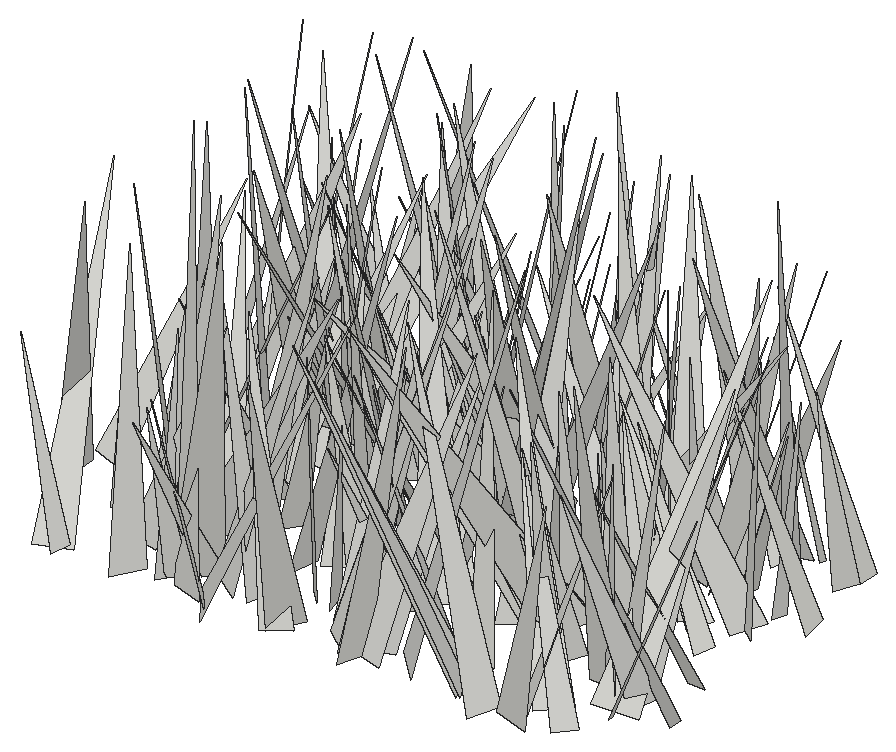
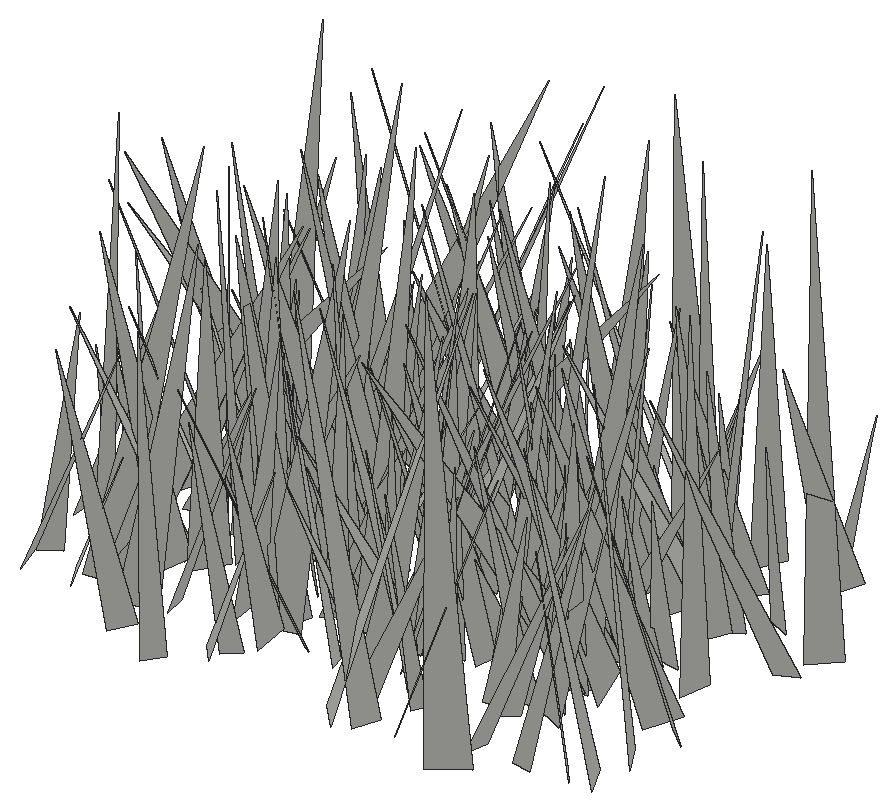
# SketchUp Ruby script. Lengths in inches.
U = 1.inch
M = Sketchup.active_model
def pt(a) = Geom::Point3d.new(a.map { |v| v * U })
def face(e, loops, mat)
  f = e.add_face(loops[0].map { |a| pt(a) })
  loops[1..].each { |l| e.add_face(l.map { |a| pt(a) }).erase! }
  f.material = f.back_material = mat if mat
  f
end
# faces: each face lists its corners as indices into pts; further lists are holes
def faces(e, pts, list, mat = nil) = list.each { |f| face(e, (f[0].is_a?(Array) ? f : [f]).map { |l| l.map { |i| pts[i] } }, mat) }
# xy, xz, yz: faces in a plane at the given z, y or x. An outline is a flat list of corners, or four numbers for a rectangle; further outlines are holes
def ring(l) = l.size == 4 ? [[l[0], l[1]], [l[2], l[1]], [l[2], l[3]], [l[0], l[3]]] : l.each_slice(2).to_a
def flat(e, list, mat, &to3) = list.each { |f| face(e, (f[0].is_a?(Array) ? f : [f]).map { |l| ring(l).map { |u, v| to3.(u, v) } }, mat) }
def xy(e, z, list, mat = nil) = flat(e, list, mat) { |x, y| [x, y, z] }
def xz(e, y, list, mat = nil) = flat(e, list, mat) { |x, z| [x, y, z] }
def yz(e, x, list, mat = nil) = flat(e, list, mat) { |y, z| [x, y, z] }
def lines(e, pts, list) = list.each { |a, b| e.add_line(pt(pts[a]), pt(pts[b])) }
# prism: a flat outline (further loops are holes) pulled along v
def prism(e, loops, v, mat = nil)
  f = face(e, loops, mat); d = Geom::Vector3d.new(v.map { |x| x * U })
  f.pushpull(f.normal.samedirection?(d) ? d.length : -d.length)
end
def box(e, o, s, mat = nil) = prism(e, [[o, [o[0] + s[0], o[1], o[2]], [o[0] + s[0], o[1] + s[1], o[2]], [o[0], o[1] + s[1], o[2]]]], [0, 0, s[2]], mat)
def at(x, y, z, deg = 0) = Geom::Transformation.translation(pt([x, y, z])) * Geom::Transformation.rotation(ORIGIN, Z_AXIS, deg.degrees)
def axes(o, x, y, z) = Geom::Transformation.new([*x, 0, *y, 0, *z, 0, *pt(o).to_a, 1])
def part(name) = M.definitions.add(name)
# library, detail: a bought-in or finely detailed component or shape, given as its bounding box
def library(name, o, s) = part(name).tap { |d| box(d.entities, o, s) }
def detail(e, o, s) = box(e.add_group.entities, o, s)
def put(e, d, t, mat = nil) = e.add_instance(d, t).tap { |i| i.material = mat if mat }
def group(e, t, mat = nil) = e.add_group.tap { |g| g.transformation = t; g.material = mat if mat }.entities
root = M.entities
c1 = part("fur_instance\#9")
p = [[0.8125,0,1.79],[0.67,-0.02,1.48],[0,-0.11,0],[0,0.11,0]]
faces(c1.entities,p,[[0,1,2,3]])
put(root,c1,axes([122.97,12.12,-27.1],[4.57924,-4.33247,0.58798],[-4.22206,-4.60304,-1.03525],[-1.13589,-0.35667,6.21836]))
put(root,c1,axes([129.89,12.79,-27.1],[-6.83596,-2.73328,0.53057],[-2.58478,6.75268,1.48423],[1.035,-1.18879,7.21098]))
put(root,c1,axes([132.79,11.72,-27.1],[0.54307,-5.39112,1.14857],[-5.29865,-0.1925,1.60174],[1.51911,1.25582,5.17624]))
put(root,c1,axes([129.98,12.7,-27.1],[-5.72076,-3.26575,0.35826],[-3.1922,5.6955,0.94426],[0.77675,-0.64548,6.51924]))
put(root,c1,axes([118.09,12.47,-27.1],[2.18541,-3.04998,0.78828],[-3.02604,-2.29919,-0.50659],[-0.87571,0.3334,3.71777]))
put(root,c1,axes([118.98,13.31,-27.1],[1.51991,-3.61395,0.26794],[-3.4425,-1.53065,-1.11749],[-1.13207,-0.1975,3.75792]))
put(root,c1,axes([113.92,11.49,-27.1],[-3.79892,0.58903,0.61511],[0.5899,3.84804,-0.04166],[0.61427,-0.05255,3.84409]))
put(root,c1,axes([126.1,11.77,-27.1],[6.14943,-1.42717,1.61929],[-1.52874,-6.3314,0.22535],[-1.52376,0.59247,6.30885]))
put(root,c1,axes([118.09,13.56,-27.1],[6.18232,-5.30847,0.7026],[-5.32058,-6.21081,-0.10875],[-0.60412,0.37485,8.14795]))
put(root,c1,axes([119.89,11.47,-27.1],[5.9079,4.20697,0.32991],[4.15488,-5.69984,-1.72033],[0.73785,-1.5887,7.04573]))
put(root,c1,axes([120.04,11.49,-27.1],[-3.12705,-1.8127,0.50032],[-1.87769,2.95706,-1.02213],[-0.10232,1.13341,3.46693]))
put(root,c1,axes([116.66,11.66,-27.1],[-5.0872,2.66073,2.45988],[2.85923,5.55214,-0.09239],[2.22604,-1.05084,5.74025]))
put(root,c1,axes([122.9,11.67,-27.1],[-2.01026,5.06538,1.49078],[5.275,1.85579,0.80751],[-0.23431,-1.67916,5.38954]))
put(root,c1,axes([131.7,11.64,-27.1],[-6.69944,1.03913,0.45559],[1.00559,6.70154,-0.49804],[0.5255,0.42362,6.76123]))
put(root,c1,axes([125.62,12.28,-27.1],[5.24089,-0.83273,1.62957],[-1.05437,-5.41429,0.62423],[-1.49573,0.89885,5.2698]))
put(root,c1,axes([126.2,12.0625,-27.1],[0.11042,6.13884,2.00494],[6.14565,0.51615,-1.91884],[1.98398,-1.94051,5.83229]))
put(root,c1,axes([111.09,15.68,-27.1],[8.00988,-2.00577,0.3429],[-1.833,-7.71682,-2.32157],[-0.88363,-2.17404,7.92412]))
put(root,c1,axes([119.03,11.81,-27.1],[2.99088,7.34321,2.70362],[7.47912,-3.53374,1.32409],[-2.30112,-1.94104,7.81761]))
put(root,c1,axes([134.58,12.33,-27.1],[-1.36293,4.52681,0.55653],[4.38086,1.13777,1.47406],[-1.26877,-0.93423,4.49185]))
put(root,c1,axes([117.8,12.125,-27.1],[-4.10668,0.43412,1.0008],[0.12519,4.05996,-1.24738],[1.0837,1.17608,3.93666]))
put(root,c1,axes([132.625,14.21,-27.1],[1.7038,-4.78318,1.39426],[-4.94528,-1.80274,-0.14134],[-0.60574,1.26373,5.0756]))
put(root,c1,axes([119.65,13,-27.1],[3.29943,5.39851,1.49465],[5.593,-3.07886,-1.22601],[0.31023,-1.9081,6.20701]))
put(root,c1,axes([133.89,15.56,-27.1],[0.64901,-7.30772,0.94418],[-7.33385,-0.54888,0.79295],[0.71332,1.00569,7.2935]))
put(root,c1,axes([132.78,12.3125,-27.1],[3.07177,3.42083,0.35758],[3.42072,-3.08846,0.16062],[-0.35863,-0.15826,4.59478]))
put(root,c1,axes([135.51,15.33,-27.1],[3.42862,-3.42654,1.21049],[-3.04602,-3.61734,-1.61199],[-1.98197,-0.36822,4.57144]))
put(root,c1,axes([127.79,12.51,-27.1],[5.42391,5.6075,1.42758],[5.74422,-5.4537,-0.40246],[-0.69711,-1.3092,7.79108]))
put(root,c1,axes([115.7,13.58,-27.1],[1.80806,-4.3936,1.6396],[-4.55829,-1.23367,1.72079],[1.10181,2.10605,4.4285]))
put(root,c1,axes([123.3,14.35,-27.1],[3.69206,0.52175,1.19179],[0.74035,-3.79133,-0.63373],[-1.0698,-0.8231,3.6745]))
put(root,c1,axes([128.84,13.87,-27.1],[-4.50374,-2.5863,0.2222],[-2.55985,4.35118,-1.23954],[-0.43072,1.18335,5.04343]))
put(root,c1,axes([130.17,17.97,-27.1],[4.91107,-6.51993,1.1851],[-5.42781,-4.80392,-3.93621],[-3.80168,-1.5638,7.15082]))
put(root,c1,axes([121.08,13.01,-27.1],[-5.72971,0.10944,0.75393],[-0.02545,5.68949,-1.01935],[0.7614,1.01378,5.63937]))
put(root,c1,axes([124.99,12.29,-27.1],[4.48947,6.23838,0.89691],[6.27438,-4.52789,0.08708],[-0.59503,-0.67674,7.68539]))
put(root,c1,axes([115.95,15.24,-27.1],[-4.21383,-5.23135,2.06774],[-5.35043,4.52497,0.54449],[1.7365,1.24763,6.69529]))
put(root,c1,axes([133.375,13.26,-27.1],[-3.60307,5.2202,0.86904],[5.28801,3.51043,0.83765],[-0.20649,-1.18922,6.28736]))
put(root,c1,axes([125.52,15.4,-27.1],[0.6602,-3.48398,0.63366],[-3.31771,-0.83389,-1.12823],[-1.23791,0.37685,3.36171]))
put(root,c1,axes([113.64,11.46,-27.1],[-5.02723,4.35262,0.08247],[4.19421,4.87628,-1.68986],[1.1665,1.22544,6.43138]))
put(root,c1,axes([122.49,14.28,-27.1],[2.78644,2.89477,1.9564],[3.12581,-3.18339,0.25829],[-1.56092,-1.20736,4.00964]))
put(root,c1,axes([124.03,15.09,-27.1],[2.18387,-4.44969,1.85832],[-4.59717,-2.53702,-0.67228],[-1.45572,1.33648,4.91091]))
put(root,c1,axes([126.52,12.7,-27.1],[-3.94538,2.89092,1.6801],[2.22143,4.20848,-2.02488],[2.49909,0.82308,4.45234]))
put(root,c1,axes([124.66,13.32,-27.1],[0.1573,5.82785,1.1486],[5.93788,-0.12389,-0.18455],[0.15705,-1.15268,5.82705]))
put(root,c1,axes([124.28,14.03,-27.1],[6.01682,-1.89651,1.60783],[-2.22,-5.99358,1.23799],[-1.11958,1.69241,6.18597]))
put(root,c1,axes([134.61,14.67,-27.1],[2.05844,3.54151,1.67651],[3.74882,-2.33096,0.32115],[-1.13989,-1.27062,4.08367]))
put(root,c1,axes([131.76,16.25,-27.1],[3.25434,-3.10316,1.28908],[-2.93626,-3.49873,-1.00964],[-1.63392,0.10675,4.38189]))
put(root,c1,axes([116.9,15.67,-27.1],[3.69144,-5.31541,0.62902],[-5.0613,-3.21782,2.51095],[1.74141,1.9152,5.96452]))
put(root,c1,axes([128.98,17.73,-27.1],[-6.06549,-1.51995,0.44377],[-1.27134,5.72216,2.22212],[0.94386,-2.06007,5.84487]))
put(root,c1,axes([137.13,14.98,-27.1],[-3.79929,-4.93063,0.76728],[-4.2284,2.66909,-3.78564],[-2.64961,2.81057,4.94112]))
put(root,c1,axes([134.55,15.44,-27.1],[2.41252,4.65389,1.89869],[5.02303,-2.30836,-0.72433],[-0.1815,-2.02404,5.19175]))
put(root,c1,axes([113.76,14.76,-27.1],[0.89714,3.83975,1.01573],[3.88067,-1.06922,0.61438],[-0.84607,-0.83267,3.89501]))
put(root,c1,axes([114.77,15.99,-27.1],[1.60896,-4.17155,1.4473],[-4.41412,-1.4813,0.63763],[0.1098,1.57772,4.42538]))
put(root,c1,axes([129.64,14.08,-27.1],[1.15539,6.15443,1.22459],[6.01284,-1.44203,1.57415],[-1.79512,-0.86897,6.06086]))
put(root,c1,axes([123.45,15.85,-27.1],[2.89079,5.81329,3.19782],[6.3896,-3.37876,0.3661],[-1.787,-2.67707,6.48205]))
put(root,c1,axes([136.08,17.4,-27.1],[-1.33885,-4.31341,0.19295],[-4.24788,1.27969,-0.86785],[-0.77346,0.43835,4.43226]))
put(root,c1,axes([130.73,17.07,-27.1],[-7.92829,-1.68885,1.19775],[-1.65667,8.01779,0.33921],[1.24187,-0.08605,8.09907]))
put(root,c1,axes([127.43,16.95,-27.1],[-4.42248,-6.55022,0.11235],[-5.68971,3.77318,-3.9833],[-3.24733,2.30957,6.8262]))
put(root,c1,axes([120.95,15.55,-27.1],[6.83211,0.09479,1.62922],[-0.11306,-6.96812,0.87954],[-1.62805,0.88169,6.77592]))
put(root,c1,axes([118.62,15.87,-27.1],[6.64236,-2.17739,2.19825],[-2.53423,-6.81539,0.90685],[-1.77512,1.5823,6.93106]))
put(root,c1,axes([122.98,18.65,-27.1],[-2.64137,-6.46023,1.04071],[-6.35863,2.79897,1.23619],[1.54452,0.47506,6.86901]))
put(root,c1,axes([124.71,17,-27.1],[-2.99975,-3.60869,1.08185],[-3.74003,3.01886,-0.30041],[0.45307,1.02732,4.68304]))
put(root,c1,axes([125.92,17.72,-27.1],[-2.72161,-4.19987,1.18368],[-4.18397,2.90781,0.69726],[1.23872,0.59401,4.95579]))
put(root,c1,axes([124.97,18.24,-27.1],[-3.4454,-3.89131,0.03074],[-3.88746,3.44363,0.20759],[0.17579,-0.11462,5.19326]))
put(root,c1,axes([115.02,16.64,-27.1],[5.24676,-2.59436,1.90695],[-2.83441,-5.4512,0.38233],[-1.5275,1.20389,5.84064]))
put(root,c1,axes([118.98,17.45,-27.1],[3.98619,-2.41358,0.43201],[-2.42835,-4.00018,0.05811],[-0.33929,0.27366,4.65958]))
put(root,c1,axes([133.05,16.31,-27.1],[-3.3024,-1.44134,1.34219],[-1.74105,3.36144,-0.674],[0.92071,1.18661,3.53964]))
put(root,c1,axes([121.53,17.41,-27.1],[-4.43723,-6.45792,2.6794],[-6.95056,4.4181,-0.86196],[0.75734,2.71083,7.78786]))
put(root,c1,axes([134.17,16.81,-27.1],[3.16186,-4.77933,2.12939],[-5.21892,-2.70344,1.68164],[0.37303,2.68757,5.47827]))
put(root,c1,axes([126.05,16.47,-27.1],[-4.29093,5.93832,1.73067],[6.14946,4.32229,0.41585],[0.66564,-1.65078,7.31456]))
put(root,c1,axes([135.22,13.9375,-27.1],[5.40862,3.75774,0.29196],[3.28966,-4.95573,2.84217],[-1.83956,2.18614,5.94103]))
put(root,c1,axes([130.49,17.97,-27.1],[3.95695,-1.9726,1.7752],[-1.97238,-4.31833,-0.40205],[-1.77544,0.40099,4.40306]))
put(root,c1,axes([126.03,17.29,-27.1],[3.90442,0.1948,1.09665],[0.0575,-4.02752,0.51071],[-1.11233,0.47558,3.87577]))
put(root,c1,axes([115.68,15.78,-27.1],[5.65943,2.62486,0.30549],[2.50558,-5.55953,1.3513],[-0.8398,1.10185,6.0904]))
put(root,c1,axes([117.69,18.8,-27.1],[-0.92246,-4.02488,0.49642],[-3.83236,0.69867,-1.45667],[-1.32631,0.78053,3.86377]))
put(root,c1,axes([132.05,18.33,-27.1],[4.08918,-3.36848,1.98263],[-3.52303,-4.41912,-0.24183],[-1.69286,1.05996,5.29241]))
put(root,c1,axes([120.55,19.63,-27.1],[2.722,-4.21365,0.18087],[-4.20663,-2.72794,-0.24377],[-0.30292,0.01939,5.01046]))
put(root,c1,axes([132.64,18.22,-27.1],[4.18709,2.7222,0.51054],[2.74144,-3.94162,-1.4666],[0.39441,-1.502,4.77401]))
put(root,c1,axes([135.03,14.38,-27.1],[-5.0261,5.87636,0.71878],[5.2638,4.86732,-2.98524],[2.70938,1.44485,7.13314]))
put(root,c1,axes([126.26,17.08,-27.1],[-4.785,3.6619,0.62252],[3.69492,4.79647,0.18627],[0.38032,-0.52686,6.02254]))
put(root,c1,axes([128.17,20.79,-27.1],[-1.4202,-8.16889,0.91065],[-8.13373,1.52988,1.03868],[1.18423,0.71114,8.22611]))
put(root,c1,axes([118.68,16.84,-27.1],[-6.74078,-2.87477,2.26806],[-3.46071,6.55422,-1.97791],[1.19661,2.76122,7.05622]))
put(root,c1,axes([125.06,18.35,-27.1],[-5.1041,-1.8904,0.52095],[-1.9461,5.06157,-0.70004],[0.24022,0.83889,5.39772]))
put(root,c1,axes([131.35,19.34,-27.1],[3.43553,-2.13589,0.95207],[-2.02418,-3.56342,-0.68999],[-1.17096,-0.10667,3.98608]))
put(root,c1,axes([121.74,16.25,-27.1],[-4.67511,2.29396,0.21165],[2.12082,4.47274,-1.63107],[0.89953,1.37696,4.94555]))
put(root,c1,axes([128.85,17,-27.1],[5.55139,-3.03279,3.66915],[-4.09539,-5.91606,1.30628],[-2.42657,3.04644,6.18946]))
put(root,c1,axes([127.66,19.56,-27.1],[-3.40896,-3.60182,1.17644],[-3.63778,3.55381,0.3393],[1.06005,0.61272,4.94762]))
put(root,c1,axes([111.49,17.15,-27.1],[0.65579,5.75921,0.77226],[5.58682,-0.41126,-1.67728],[1.5976,-0.92592,5.54845]))
put(root,c1,axes([122.79,16.96,-27.1],[3.66563,6.83822,1.35122],[6.90712,-3.76874,0.33492],[-0.93742,-1.02919,7.75151]))
put(root,c1,axes([123.39,23.41,-27.1],[-6.54697,-3.05595,0.68846],[-2.14459,5.53525,4.1758],[2.28332,-3.56338,5.89613]))
put(root,c1,axes([116.68,18.9,-27.1],[2.49544,-4.2024,1.5625],[-4.46283,-2.15679,1.32672],[0.42981,2.0042,4.70396]))
put(root,c1,axes([119.15,20.29,-27.1],[4.7247,0.27251,1.48983],[0.66278,-4.76043,-1.23114],[-1.36183,-1.37139,4.56961]))
put(root,c1,axes([113.26,19.82,-27.1],[6.40054,-0.55178,2.21578],[-0.37829,-6.75939,-0.5905],[-2.25189,-0.43282,6.39709]))
put(root,c1,axes([116.55,22.1,-27.1],[2.6634,-7.09113,0.13913],[-7.08626,-2.66678,-0.26525],[-0.29724,0.03689,7.57017]))
put(root,c1,axes([132.38,19.14,-27.1],[-1.64307,3.38565,0.94063],[3.51296,1.55882,0.52563],[-0.08077,-1.0745,3.72639]))
put(root,c1,axes([134.79,19.41,-27.1],[-3.98782,0.86871,0.11292],[0.87287,3.98492,0.16912],[0.07423,-0.18933,4.07783]))
put(root,c1,axes([125.3,21.63,-27.1],[4.0127,-3.86264,0.72099],[-3.71726,-4.06564,-1.09277],[-1.27351,-0.30356,5.46147]))
put(root,c1,axes([119.8,20.89,-27.1],[-1.12963,-3.6746,0.26296],[-3.62855,1.06225,-0.74377],[-0.63679,0.46567,3.77168]))
put(root,c1,axes([125.83,23.48,-27.1],[-6.83742,-2.67371,1.15288],[-1.91772,6.34944,3.35188],[2.19094,-2.7864,6.53176]))
put(root,c1,axes([123.98,23.41,-27.1],[7.80685,-2.34529,0.78759],[-1.91376,-7.37702,-2.99744],[-1.56786,-2.67335,7.58041]))
put(root,c1,axes([115.52,19.2,-27.1],[0.0321,3.78164,0.61426],[3.82721,-0.05969,0.16749],[-0.17489,-0.6122,3.77806]))
put(root,c1,axes([129.6,18.16,-27.1],[5.08694,2.79276,1.06084],[2.31416,-5.00849,2.08845],[-1.88933,1.38471,5.41433]))
put(root,c1,axes([122.38,22.26,-27.1],[-4.64993,-4.92524,0.42817],[-4.93518,4.6591,-0.00251],[0.29211,0.31306,6.77347]))
put(root,c1,axes([135.03,21.47,-27.1],[-3.6368,4.97548,2.15784],[5.29036,2.68314,2.72961],[-1.1932,-3.26854,5.52548]))
put(root,c1,axes([133.67,20.63,-27.1],[-3.19624,2.75407,0.40141],[2.73336,2.9911,1.24258],[-0.52417,-1.19599,4.03198]))
put(root,c1,axes([115.23,18.95,-27.1],[-0.56854,4.75375,0.07359],[4.64609,0.5398,1.02436],[-1.0087,-0.19303,4.67676]))
put(root,c1,axes([131.26,22,-27.1],[-4.22534,-4.50008,2.6097],[-4.33201,4.90527,1.44456],[2.88009,0.77613,6.00146]))
put(root,c1,axes([126.45,20.7,-27.1],[6.91635,-1.96319,0.7746],[-2.05636,-6.86586,0.95992],[-0.47486,1.1384,7.12521]))
put(root,c1,axes([125.375,20.28,-27.1],[7.84011,2.17766,1.89393],[2.14429,-8.06482,0.39652],[-1.93163,-0.114,8.12726]))
put(root,c1,axes([126.08,20.98,-27.1],[-4.47703,-2.46915,0.00102],[-2.34184,4.24552,-1.62229],[-0.78262,1.42103,4.84857]))
put(root,c1,axes([117.35,21.2,-27.1],[5.44742,2.57642,1.57153],[2.74581,-5.57692,-0.37485],[-1.25227,-1.0208,6.0143]))
put(root,c1,axes([131.55,20.27,-27.1],[-7.28379,2.71503,1.56111],[2.64145,7.44897,-0.63058],[1.68261,0.05921,7.74773]))
put(root,c1,axes([130.53,22.14,-27.1],[5.81902,2.09502,1.94943],[2.48849,-5.88572,-1.1028],[-1.4131,-1.7377,6.08555]))
put(root,c1,axes([121.86,20.8,-27.1],[0.71871,3.7725,0.80138],[3.83913,-0.62217,-0.51422],[0.36739,-0.87844,3.80576]))
put(root,c1,axes([135.17,21.18,-27.1],[2.79154,3.79561,1.789],[3.98615,-3.06992,0.29332],[-1.31064,-1.25251,4.70248]))
put(root,c1,axes([116.65,19.84,-27.1],[1.55452,5.85258,0.28483],[5.77094,-1.47817,-1.12324],[1.01494,-0.55917,5.95042]))
put(root,c1,axes([124.1,22.3125,-27.1],[0.22689,-3.51122,0.97081],[-3.62685,-0.12635,0.39066],[0.3422,0.98893,3.49679]))
put(root,c1,axes([130.54,21.01,-27.1],[-2.56552,5.11443,0.44811],[4.78646,2.20153,2.27666],[-1.85689,-1.39139,5.24939]))
put(root,c1,axes([122.05,21.4,-27.1],[2.7927,4.03544,0.85961],[4.11922,-2.66751,-0.85986],[0.23622,-1.19268,4.83163]))
put(root,c1,axes([118.55,23.47,-27.1],[-2.6676,-6.3456,1.58153],[-6.4273,2.85927,0.63121],[1.20736,1.20081,6.85451]))
put(root,c1,axes([133.08,20.82,-27.1],[-0.96186,4.58475,0.31518],[4.19254,0.74357,1.97843],[-1.88199,-0.68675,4.24628]))
put(root,c1,axes([131.32,19.25,-27.1],[-7.41355,2.38035,1.13819],[1.92535,7.2016,-2.52036],[1.80404,2.09598,7.36713]))
put(root,c1,axes([136.68,22.87,-27.1],[-4.93591,-0.64757,0.62999],[-0.58328,4.95621,0.52453],[0.68994,-0.44273,4.95049]))
put(root,c1,axes([133.66,21.89,-27.1],[1.6531,3.56586,0.9383],[3.65871,-1.45863,-0.90264],[0.45784,-1.21883,3.82535]))
put(root,c1,axes([119.42,21.6,-27.1],[-0.23432,4.6061,1.3303],[4.44797,-0.2882,1.78136],[-1.78924,-1.31967,4.25416]))
put(root,c1,axes([128.08,23.61,-27.1],[5.88193,4.68919,0.48239],[4.10623,-4.71789,-4.20698],[2.31519,-3.54559,6.23594]))
put(root,c1,axes([122.81,22.53,-27.1],[-3.89073,-0.42692,0.42553],[-0.44504,3.90915,-0.14719],[0.40654,0.19356,3.91132]))
put(root,c1,axes([131.64,23.01,-27.1],[-0.96334,-4.21277,1.52504],[-4.43315,1.12201,0.29911],[0.64835,1.41239,4.31115]))
put(root,c1,axes([129.72,21.65,-27.1],[-5.3119,3.70536,1.5571],[3.75007,5.49761,-0.28937],[1.44609,-0.64586,6.4701]))
put(root,c1,axes([127.46,22.09,-27.1],[-4.33935,-4.28478,3.74469],[-5.00881,5.11096,0.04388],[2.70071,2.59437,6.09815]))
put(root,c1,axes([132.02,21.24,-27.1],[3.70568,3.40586,0.49894],[3.35111,-3.73706,0.62078],[-0.78668,0.12425,4.99466]))
put(root,c1,axes([115.99,24.19,-27.1],[-2.53564,-6.45433,1.27855],[-6.57975,2.48748,-0.49186],[0.00081,1.3699,6.91708]))
put(root,c1,axes([133.48,23.34,-27.1],[3.83276,-0.80553,0.30542],[-0.78769,-3.84079,-0.24507],[-0.34886,-0.17786,3.90882]))
put(root,c1,axes([118.94,22.06,-27.1],[0.50211,5.33526,1.29674],[5.04367,0.06639,-2.22613],[2.16978,-1.38897,4.87457]))
put(root,c1,axes([112.73,22.15,-27.1],[4.48664,-4.30175,1.96808],[-4.72578,-3.95369,2.13158],[0.21294,2.89338,5.83878]))
put(root,c1,axes([126.22,21.52,-27.1],[-6.64988,-1.58039,2.79885],[-2.32051,6.81074,-1.66765],[2.22405,2.38079,6.62853]))
put(root,c1,axes([126.61,25.14,-27.1],[2.5513,-6.67742,1.15565],[-6.68995,-2.67869,-0.70836],[-1.08074,0.81812,7.11304]))
put(root,c1,axes([133.07,26.18,-27.1],[1.39715,-7.46285,0.32526],[-7.45597,-1.41344,-0.40331],[-0.45656,0.24497,7.58179]))
put(root,c1,axes([135.3,22.74,-27.1],[-3.53887,0.08812,1.47041],[-0.2173,3.75324,-0.74791],[1.45693,0.77383,3.46005]))
put(root,c1,axes([119.8125,22.21,-27.1],[-4.5359,3.17744,2.60533],[2.766,5.23085,-1.56386],[3.0386,-0.01843,5.3127]))
put(root,c1,axes([121.87,24.35,-27.1],[-4.72321,-4.87597,2.05821],[-5.0831,4.94763,0.05633],[1.47426,1.43735,6.78828]))
put(root,c1,axes([111.76,22.64,-27.1],[3.62165,4.35293,0.90177],[4.41878,-3.65214,-0.11732],[-0.48531,-0.76904,5.66132]))
put(root,c1,axes([121.12,23.23,-27.1],[-2.98056,5.41129,1.99239],[5.72855,3.03527,0.32601],[0.65987,-1.90801,6.16924]))
put(root,c1,axes([134.3125,24.69,-27.1],[3.79237,5.90894,3.79832],[6.9076,-3.92109,-0.79686],[-1.27587,-3.6653,6.97586]))
put(root,c1,axes([122.59,23.3125,-27.1],[-0.71726,5.0627,1.58469],[5.02661,0.13746,1.836],[-1.69568,-1.73401,4.77227]))
put(root,c1,axes([116.52,22.26,-27.1],[2.2285,7.10603,0.93052],[7.02267,-1.97084,-1.76797],[1.42959,-1.39565,7.23438]))
put(root,c1,axes([116.18,23.19,-27.1],[2.91004,3.86675,2.0314],[3.84438,-3.42612,1.0144],[-2.0734,-0.92551,4.73192]))
put(root,c1,axes([126.39,24.55,-27.1],[6.40795,-1.734,1.03011],[-1.73088,-6.48917,-0.15614],[-1.03535,0.11648,6.63658]))
put(root,c1,axes([115.55,21.48,-27.1],[-6.44163,0.17845,3.84936],[-1.24896,6.99677,-2.4144],[3.64548,2.71245,5.9747]))
put(root,c1,axes([116.66,22.3125,-27.1],[-2.09458,6.39775,0.76013],[6.40195,1.97698,1.00139],[-0.72385,-1.02792,6.657]))
put(root,c1,axes([122.02,24.02,-27.1],[-7.0839,-2.86843,1.00142],[-2.98784,7.03787,-0.97651],[0.55097,1.28563,7.57997]))
put(root,c1,axes([116.6875,21.21,-27.1],[-2.61013,7.00123,1.33294],[6.01827,2.92557,-3.58165],[3.81765,0.17478,6.55758]))
put(root,c1,axes([131.94,23.95,-27.1],[5.79665,-1.91222,1.6292],[-2.17494,-5.87047,0.84811],[-1.25719,1.33905,6.04471]))
put(root,c1,axes([116.87,23.98,-27.1],[0.82444,4.69785,1.50621],[4.90559,-0.61872,-0.75536],[0.52313,-1.60174,4.70945]))
put(root,c1,axes([130.95,23.34,-27.1],[-5.28353,4.19242,1.51467],[4.2139,5.46353,-0.42331],[1.45386,-0.59977,6.73148]))
put(root,c1,axes([122.89,24.47,-27.1],[-6.49588,1.72746,1.45223],[1.82521,6.62397,0.28488],[1.32729,-0.65455,6.71561]))
put(root,c1,axes([124.64,22.97,-27.1],[3.32895,2.2471,0.95718],[1.81279,-3.35751,1.57751],[-1.63691,0.85163,3.69362]))
put(root,c1,axes([125.71,23.1,-27.1],[1.80048,6.74236,1.9451],[6.61582,-2.30046,1.85022],[-2.33959,-1.31645,6.72888]))
put(root,c1,axes([122.62,22.75,-27.1],[4.4552,2.25801,0.37031],[2.04407,-4.29173,1.57715],[-1.02836,1.2518,4.7392]))
put(root,c1,axes([135.78,25.7,-27.1],[3.23004,-2.47849,1.2151],[-2.38486,-3.44753,-0.69249],[-1.3899,0.15559,4.01205]))
put(root,c1,axes([111.95,24.72,-27.1],[5.69134,3.55142,2.30083],[3.82093,-5.97012,-0.23634],[-1.81848,-1.42926,6.70433]))
put(root,c1,axes([132.38,22.75,-27.1],[4.78963,3.34115,0.62659],[3.09789,-4.73577,1.57225],[-1.39963,0.95165,5.62422]))
put(root,c1,axes([123.64,25.72,-27.1],[4.61843,1.91697,0.98697],[2.11588,-4.47821,-1.2031],[-0.41467,-1.49987,4.85358]))
put(root,c1,axes([117.01,24.99,-27.1],[-3.73085,2.02538,0.45172],[2.07172,3.68874,0.57157],[0.11914,-0.71871,4.20651]))
put(root,c1,axes([117.73,24.68,-27.1],[-1.66438,3.94539,0.96796],[4.04045,1.49913,0.83702],[-0.42169,-1.20819,4.19948]))
put(root,c1,axes([120.79,25.46,-27.1],[3.65523,2.01923,0.98653],[2.16689,-3.66612,-0.52479],[-0.59594,-0.94526,4.14277]))
put(root,c1,axes([121.82,24.01,-27.1],[6.24718,3.3719,1.68528],[3.2403,-6.4703,0.93425],[-1.92623,0.05148,7.03734]))
put(root,c1,axes([114.52,27.39,-27.1],[-1.82022,-4.66244,0.24993],[-4.60062,1.83672,0.75812],[0.79693,-0.04591,4.9474]))
put(root,c1,axes([130.1875,26.08,-27.1],[-4.58656,-0.99691,0.53395],[-0.9871,4.61746,0.14195],[0.55187,-0.02624,4.69151]))
put(root,c1,axes([119.61,26.43,-27.1],[3.62629,-0.3933,0.08931],[-0.3696,-3.56406,-0.68808],[-0.16141,-0.67481,3.58206]))
put(root,c1,axes([133.125,25.64,-27.1],[-3.66432,1.46778,0.50332],[1.5223,3.65057,0.437],[0.30055,-0.59495,3.9231]))
put(root,c1,axes([131.15,26.85,-27.1],[1.6386,-6.2759,2.07036],[-6.47654,-1.94928,-0.78297],[-1.31443,1.78093,6.43885]))
put(root,c1,axes([125.04,25.59,-27.1],[3.37481,3.69249,0.11879],[3.55193,-3.19874,-1.47981],[1.01606,-1.08238,4.77849]))
put(root,c1,axes([121.48,27.01,-27.1],[-0.67131,-4.1889,0.93111],[-4.10147,0.34927,-1.38579],[-1.26165,1.09345,4.00962]))
put(root,c1,axes([119.22,28.09,-27.1],[-4.05728,-2.523,0.42943],[-2.40041,4.03064,1.00168],[0.88766,-0.63233,4.67158]))
put(root,c1,axes([128.2,24.62,-27.1],[-7.28792,0.99409,0.70676],[0.80322,7.1337,-1.75122],[0.9179,1.65037,7.1439]))
put(root,c1,axes([121.63,28.6875,-27.1],[-5.81753,-5.50464,0.89808],[-5.45533,5.88597,0.73893],[1.16061,0.07452,7.97488]))
put(root,c1,axes([124.1,24.13,-27.1],[3.59429,3.23742,0.8797],[2.57384,-3.488,2.32011],[-2.15177,1.23558,4.24464]))
put(root,c1,axes([117.62,27.5,-27.1],[4.3427,-1.50818,1.19732],[-1.3579,-4.49272,-0.73402],[-1.36538,-0.32877,4.53816]))
put(root,c1,axes([116.46,27.33,-27.1],[-5.398,0.07669,0.31538],[0.11355,5.36878,0.63804],[0.30406,-0.64352,5.36071]))
put(root,c1,axes([120.31,28.33,-27.1],[7.393,0.04175,0.28729],[0.1077,-7.1937,-1.72622],[-0.26959,-1.72907,7.18877]))
put(root,c1,axes([135.98,26.6,-27.1],[-5.12979,-1.0122,0.11272],[-1.018,5.07872,-0.72273],[-0.03042,0.73083,5.17851]))
put(root,c1,axes([116.33,28.99,-27.1],[2.3597,-7.64104,0.82634],[-7.58316,-2.17409,1.55097],[1.25061,1.23463,7.84527]))
put(root,c1,axes([112.96,26.85,-27.1],[3.09566,2.75124,1.27433],[2.88928,-3.22895,-0.04754],[-0.91941,-0.88367,4.14127]))
put(root,c1,axes([112.03,26.57,-27.1],[5.547,2.87669,1.51326],[2.93945,-5.71712,0.09337],[-1.38744,-0.61131,6.24786]))
put(root,c1,axes([126.76,27.37,-27.1],[-0.37702,3.57753,2.02822],[3.88687,0.97529,-0.99777],[1.34335,-1.81786,3.4562]))
put(root,c1,axes([134.09,26.54,-27.1],[-3.59352,-1.36236,0.30323],[-1.35819,3.22059,-1.62619],[-0.32136,1.6227,3.48208]))
put(root,c1,axes([127.36,27.87,-27.1],[-2.83398,-2.56318,0.53676],[-2.6174,2.79801,-0.45803],[0.08496,0.70049,3.79362]))
put(root,c1,axes([130.67,28.25,-27.1],[3.4493,-3.36014,0.02886],[-3.29462,-3.37365,0.97621],[0.66096,0.719,4.71542]))
put(root,c1,axes([128.57,29.27,-27.1],[5.40312,-1.02873,0.51523],[-0.87968,-5.28821,-1.33359],[-0.74156,-1.2223,5.33606]))
put(root,c1,axes([126.33,25.86,-27.1],[-5.21181,1.32812,1.31914],[0.83689,5.14396,-1.87252],[1.67442,1.56295,5.04188]))
